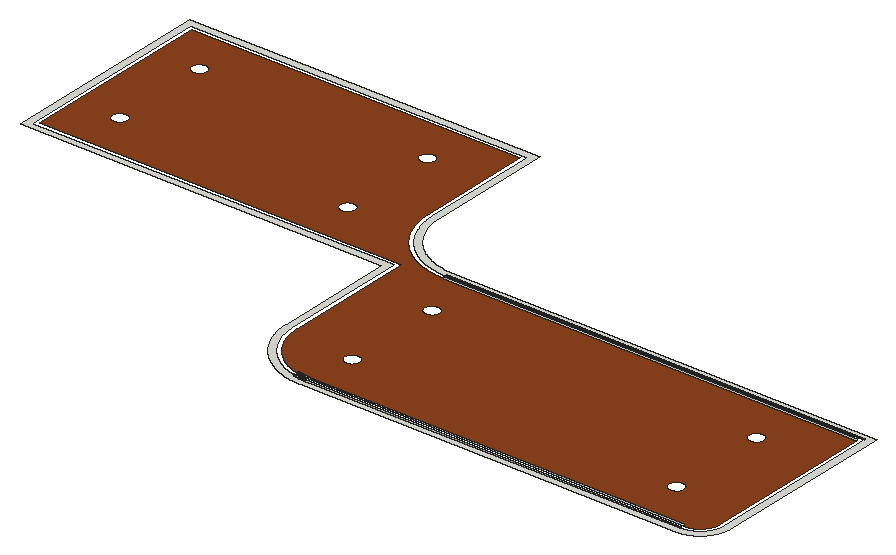
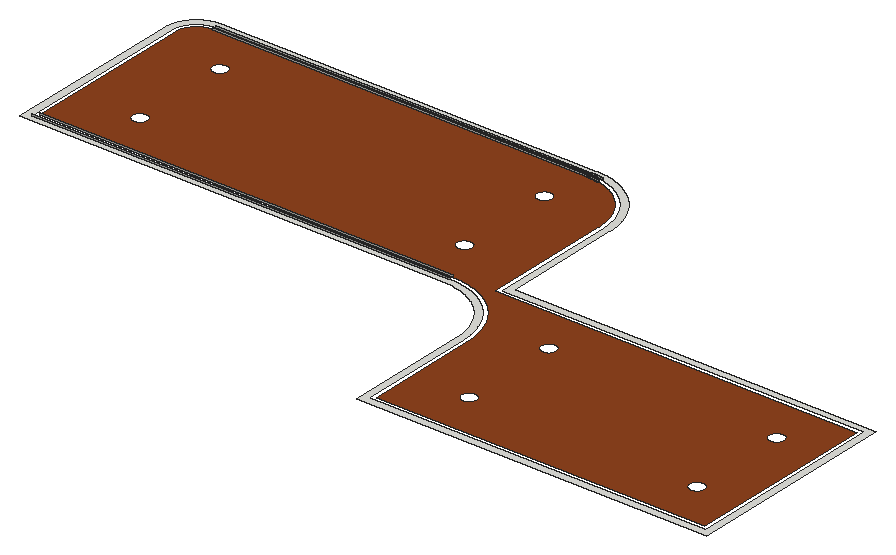
# SketchUp Ruby script. Lengths in inches.
U = 1.inch
M = Sketchup.active_model
def pt(a) = Geom::Point3d.new(a.map { |v| v * U })
def face(e, loops, mat)
  f = e.add_face(loops[0].map { |a| pt(a) })
  loops[1..].each { |l| e.add_face(l.map { |a| pt(a) }).erase! }
  f.material = f.back_material = mat if mat
  f
end
# faces: each face lists its corners as indices into pts; further lists are holes
def faces(e, pts, list, mat = nil) = list.each { |f| face(e, (f[0].is_a?(Array) ? f : [f]).map { |l| l.map { |i| pts[i] } }, mat) }
# xy, xz, yz: faces in a plane at the given z, y or x. An outline is a flat list of corners, or four numbers for a rectangle; further outlines are holes
def ring(l) = l.size == 4 ? [[l[0], l[1]], [l[2], l[1]], [l[2], l[3]], [l[0], l[3]]] : l.each_slice(2).to_a
def flat(e, list, mat, &to3) = list.each { |f| face(e, (f[0].is_a?(Array) ? f : [f]).map { |l| ring(l).map { |u, v| to3.(u, v) } }, mat) }
def xy(e, z, list, mat = nil) = flat(e, list, mat) { |x, y| [x, y, z] }
def xz(e, y, list, mat = nil) = flat(e, list, mat) { |x, z| [x, y, z] }
def yz(e, x, list, mat = nil) = flat(e, list, mat) { |y, z| [x, y, z] }
def lines(e, pts, list) = list.each { |a, b| e.add_line(pt(pts[a]), pt(pts[b])) }
# prism: a flat outline (further loops are holes) pulled along v
def prism(e, loops, v, mat = nil)
  f = face(e, loops, mat); d = Geom::Vector3d.new(v.map { |x| x * U })
  f.pushpull(f.normal.samedirection?(d) ? d.length : -d.length)
end
def box(e, o, s, mat = nil) = prism(e, [[o, [o[0] + s[0], o[1], o[2]], [o[0] + s[0], o[1] + s[1], o[2]], [o[0], o[1] + s[1], o[2]]]], [0, 0, s[2]], mat)
def at(x, y, z, deg = 0) = Geom::Transformation.translation(pt([x, y, z])) * Geom::Transformation.rotation(ORIGIN, Z_AXIS, deg.degrees)
def axes(o, x, y, z) = Geom::Transformation.new([*x, 0, *y, 0, *z, 0, *pt(o).to_a, 1])
def part(name) = M.definitions.add(name)
# library, detail: a bought-in or finely detailed component or shape, given as its bounding box
def library(name, o, s) = part(name).tap { |d| box(d.entities, o, s) }
def detail(e, o, s) = box(e.add_group.entities, o, s)
def put(e, d, t, mat = nil) = e.add_instance(d, t).tap { |i| i.material = mat if mat }
def group(e, t, mat = nil) = e.add_group.tap { |g| g.transformation = t; g.material = mat if mat }.entities
root = M.entities
M.materials.add("[Wood Fence]").color = [142, 67, 30]
xy(root,116,[[[157.71,122,157.42,122.01,157.14,122.02,156.85,122.03,156.5625,122.05,156.27,122.07,155.99,122.09,155.41,122.15,155.13,122.1875,154.84,122.23,154.56,122.27,154.27,122.32,153.71,122.42,153.43,122.48,153.14,122.54,152.58,122.68,152.31,122.75,151.75,122.91,151.48,122.99,151.2,123.08,150.66,123.26,150.12,123.46,149.85,123.57,149.58,123.67,149.32,123.79,149.05,123.9,148.53,124.14,148.01,124.4,147.76,124.53,147.5,124.67,146.75,125.09,146.51,125.24,146.26,125.39,145.3,126.03,144.84,126.37,144.61,126.55,144.38,126.72,144.15,126.9,143.93,127.09,143.71,127.27,143.49,127.46,143.07,127.84,142.44,128.44,141.84,129.07,141.46,129.49,141.27,129.71,141.09,129.93,140.9,130.15,140.72,130.38,140.55,130.61,140.37,130.84,140.03,131.3,139.39,132.26,139.24,132.51,139.09,132.75,138.67,133.5,138.53,133.76,138.4,134.01,138.14,134.53,137.9,135.05,137.79,135.32,137.67,135.58,137.57,135.85,137.46,136.12,137.26,136.66,137.08,137.2,136.99,137.48,136.91,137.75,136.75,138.31,136.68,138.58,136.54,139.14,136.48,139.43,136.42,139.71,136.32,140.27,136.27,140.56,136.23,140.84,136.1875,141.13,136.15,141.41,136.09,141.99,136.07,142.27,136.05,142.5625,136.03,142.85,136.02,143.14,136.01,143.42,136,143.71,136,182,20,182,20,250,132,250,132,209.76,132.01,209.52,132.01,209.28,132.02,209.03,132.04,208.79,132.05,208.55,132.09,208.07,132.21,207.11,132.33,206.39,132.37,206.16,132.47,205.68,132.52,205.45,132.58,205.21,132.7,204.75,132.77,204.51,133.05,203.59,133.13,203.36,133.22,203.13,133.3,202.91,133.39,202.68,133.48,202.46,133.57,202.23,133.66,202.01,133.86,201.57,133.97,201.35,134.07,201.14,134.18,200.92,134.29,200.71,134.4,200.49,134.88,199.65,135.01,199.45,135.14,199.24,135.4,198.84,135.82,198.24,135.96,198.05,136.71,197.1,137.35,196.38,137.52,196.2,137.6875,196.03,137.86,195.86,138.03,195.6875,138.2,195.52,138.38,195.35,139.1,194.71,140.05,193.96,140.24,193.82,140.84,193.4,141.24,193.14,141.45,193.01,141.65,192.88,142.49,192.4,142.71,192.29,142.92,192.18,143.14,192.07,143.35,191.97,143.57,191.86,144.01,191.66,144.23,191.57,144.46,191.48,144.68,191.39,144.91,191.3,145.13,191.22,145.36,191.13,145.59,191.05,146.51,190.77,146.75,190.7,147.21,190.58,147.45,190.52,147.68,190.47,148.16,190.37,148.39,190.33,149.11,190.21,150.07,190.09,150.55,190.05,150.79,190.04,151.03,190.02,151.28,190.01,151.52,190.01,151.76,190,288,190,288,131.8,287.99,131.61,287.98,131.41,287.97,131.22,287.93,130.82,287.91,130.63,287.875,130.4375,287.84,130.24,287.81,130.05,287.77,129.86,287.72,129.67,287.68,129.48,287.57,129.1,287.45,128.72,287.38,128.54,287.3125,128.36,287.24,128.17,287.16,127.99,287.08,127.8125,287,127.64,286.91,127.46,286.82,127.29,286.72,127.11,286.63,126.94,286.53,126.78,286.31,126.44,286.09,126.12,285.97,125.96,285.73,125.66,285.34,125.21,285.21,125.07,284.93,124.79,284.79,124.66,284.64,124.52,284.49,124.4,284.34,124.27,284.04,124.03,283.88,123.91,283.56,123.69,283.22,123.47,283.06,123.37,282.89,123.28,282.71,123.18,282.54,123.09,282.36,123,282.1875,122.92,282.01,122.84,281.83,122.76,281.64,122.6875,281.46,122.62,281.28,122.55,280.9,122.43,280.52,122.32,280.33,122.28,280.14,122.23,279.95,122.19,279.76,122.16,279.5625,122.125,279.37,122.09,279.18,122.07,278.78,122.03,278.59,122.02,278.39,122.01,278.2,122],[157.74,124,278.16,124,278.3125,124.01,278.47,124.01,278.63,124.02,278.78,124.04,279.1,124.08,279.25,124.1,279.41,124.125,279.5625,124.15,279.71,124.1875,279.87,124.22,280.32,124.34,280.77,124.49,280.92,124.55,281.0625,124.61,281.21,124.67,281.35,124.73,281.77,124.94,282.05,125.1,282.18,125.18,282.3125,125.26,282.44,125.35,282.57,125.4375,282.7,125.53,282.83,125.62,282.95,125.72,283.08,125.82,283.2,125.92,283.3125,126.02,283.43,126.125,283.54,126.23,283.66,126.34,283.77,126.46,283.875,126.57,283.98,126.6875,284.08,126.8,284.18,126.92,284.28,127.05,284.38,127.17,284.47,127.3,284.5625,127.43,284.65,127.56,284.74,127.6875,284.82,127.82,284.9,127.95,285.06,128.23,285.27,128.65,285.33,128.79,285.39,128.9375,285.45,129.08,285.51,129.23,285.66,129.68,285.78,130.13,285.8125,130.29,285.85,130.4375,285.875,130.59,285.9,130.75,285.92,130.9,285.96,131.22,285.98,131.37,285.99,131.53,285.99,131.6875,286,131.84,286,188,151.73,188,151.47,188.01,151.2,188.01,150.9375,188.03,150.67,188.04,150.41,188.06,150.14,188.08,149.875,188.1,149.61,188.13,149.35,188.16,149.08,188.19,148.56,188.27,148.3,188.3125,148.03,188.36,147.51,188.46,146.99,188.58,146.74,188.64,146.48,188.7,145.96,188.84,145.71,188.92,145.45,189,144.95,189.16,144.2,189.43,143.95,189.53,143.7,189.625,143.46,189.73,143.21,189.83,142.97,189.9375,142.73,190.05,142.49,190.16,142.01,190.4,141.78,190.52,141.54,190.64,141.08,190.9,140.85,191.04,140.62,191.17,140.39,191.3125,140.17,191.45,139.94,191.6,139.72,191.74,139.5,191.89,139.28,192.05,139.07,192.2,138.85,192.36,138.43,192.68,138.22,192.85,138.02,193.01,137.8125,193.18,137.61,193.36,137.41,193.53,137.21,193.71,137.02,193.89,136.82,194.07,136.63,194.26,136.44,194.44,136.26,194.63,136.07,194.82,135.89,195.02,135.71,195.21,135.53,195.41,135.36,195.61,135.18,195.8125,135.01,196.02,134.85,196.22,134.68,196.43,134.36,196.85,134.2,197.07,134.05,197.28,133.89,197.5,133.74,197.72,133.6,197.94,133.45,198.17,133.3125,198.39,133.17,198.62,133.04,198.85,132.9,199.08,132.64,199.54,132.52,199.78,132.4,200.01,132.16,200.49,132.05,200.73,131.9375,200.97,131.83,201.21,131.73,201.46,131.625,201.7,131.53,201.95,131.43,202.2,131.16,202.95,131,203.45,130.92,203.71,130.84,203.96,130.7,204.48,130.64,204.74,130.58,204.99,130.46,205.51,130.36,206.03,130.3125,206.3,130.27,206.56,130.19,207.08,130.16,207.35,130.13,207.61,130.1,207.875,130.08,208.14,130.06,208.41,130.04,208.67,130.03,208.9375,130.01,209.2,130.01,209.47,130,209.73,130,248,22,248,22,184,138,184,138,143.74,138.01,143.48,138.02,143.21,138.04,142.69,138.0625,142.43,138.08,142.17,138.17,141.39,138.29,140.61,138.33,140.36,138.38,140.1,138.4375,139.84,138.49,139.59,138.55,139.33,138.62,139.08,138.68,138.82,138.82,138.32,138.98,137.82,139.0625,137.57,139.15,137.32,139.24,137.08,139.33,136.83,139.42,136.59,139.52,136.35,139.73,135.87,139.84,135.625,139.95,135.39,140.0625,135.15,140.18,134.92,140.3,134.6875,140.42,134.46,140.68,134,140.8125,133.77,140.95,133.55,141.37,132.89,141.52,132.67,141.67,132.46,141.82,132.24,141.97,132.03,142.13,131.82,142.29,131.62,142.46,131.41,142.79,131.01,142.96,130.8125,143.14,130.62,143.3125,130.42,143.49,130.23,143.67,130.04,143.86,129.86,144.04,129.67,144.23,129.49,144.42,129.3125,144.62,129.14,144.8125,128.96,145.01,128.79,145.41,128.46,145.62,128.29,145.82,128.13,146.03,127.97,146.24,127.82,146.46,127.67,146.67,127.52,146.89,127.37,147.55,126.95,147.77,126.8125,148,126.68,148.46,126.42,148.6875,126.3,148.92,126.18,149.15,126.0625,149.39,125.95,149.625,125.84,149.87,125.73,150.35,125.52,150.59,125.42,150.83,125.33,151.08,125.24,151.32,125.15,151.57,125.0625,151.82,124.98,152.32,124.82,152.82,124.68,153.08,124.62,153.33,124.55,153.59,124.49,153.84,124.4375,154.1,124.38,154.36,124.33,154.61,124.29,155.39,124.17,156.17,124.08,156.43,124.0625,156.69,124.04,157.21,124.02,157.48,124.01]]])
xy(root,116,[[[157.76,125.5,157.52,125.51,157.27,125.51,157.03,125.53,156.79,125.54,156.07,125.6,155.35,125.69,154.63,125.81,154.39,125.86,154.15,125.9,153.92,125.96,153.68,126.01,153.45,126.07,153.21,126.13,152.98,126.19,152.75,126.26,152.51,126.33,152.28,126.41,152.05,126.48,151.82,126.5625,151.6,126.64,151.14,126.82,150.7,127,150.48,127.1,150.25,127.2,150.04,127.3,149.6,127.52,149.39,127.63,149.17,127.74,148.54,128.1,148.33,128.23,148.13,128.35,147.92,128.48,147.72,128.62,147.52,128.75,147.32,128.89,147.125,129.03,146.93,129.18,146.74,129.32,146.36,129.62,146.17,129.78,145.99,129.93,145.8,130.09,145.62,130.25,145.44,130.42,145.27,130.58,145.09,130.75,144.75,131.09,144.58,131.27,144.42,131.44,144.25,131.62,144.09,131.8,143.93,131.99,143.78,132.17,143.62,132.36,143.32,132.74,143.18,132.93,143.03,133.125,142.89,133.32,142.75,133.52,142.62,133.72,142.48,133.92,142.35,134.13,142.23,134.33,142.1,134.54,141.74,135.17,141.63,135.39,141.52,135.6,141.3,136.04,141.2,136.25,141.1,136.48,141,136.7,140.82,137.14,140.64,137.6,140.5625,137.82,140.48,138.05,140.41,138.28,140.33,138.51,140.26,138.75,140.19,138.98,140.13,139.21,140.07,139.45,140.01,139.68,139.96,139.92,139.9,140.15,139.86,140.39,139.81,140.63,139.69,141.35,139.6,142.07,139.54,142.79,139.53,143.03,139.51,143.27,139.51,143.52,139.5,143.76,139.5,185.5,23.5,185.5,23.5,246.5,128.5,246.5,128.5,209.72,128.51,209.43,128.52,209.15,128.53,208.86,128.54,208.58,128.5625,208.3,128.58,208.01,128.67,207.17,128.71,206.89,128.75,206.6,128.79,206.32,128.84,206.04,128.88,205.76,128.9375,205.49,128.99,205.21,129.05,204.93,129.12,204.65,129.18,204.375,129.25,204.1,129.33,203.83,129.4,203.55,129.48,203.28,129.5625,203.01,129.65,202.74,129.83,202.2,129.93,201.93,130.03,201.67,130.13,201.4,130.23,201.14,130.34,200.875,130.46,200.61,130.57,200.36,130.6875,200.1,130.81,199.84,130.93,199.58,131.0625,199.33,131.19,199.08,131.33,198.83,131.46,198.58,131.6,198.33,131.74,198.09,131.89,197.84,132.04,197.6,132.1875,197.36,132.34,197.12,132.5,196.89,132.66,196.65,132.82,196.42,132.99,196.1875,133.16,195.96,133.33,195.73,133.5,195.51,133.68,195.28,133.86,195.0625,134.04,194.85,134.22,194.63,134.79,194,134.99,193.79,135.18,193.58,135.58,193.18,135.79,192.99,136,192.79,136.63,192.22,136.85,192.04,137.0625,191.86,137.28,191.68,137.51,191.5,137.73,191.33,137.96,191.16,138.1875,190.99,138.42,190.82,138.65,190.66,138.89,190.5,139.12,190.34,139.36,190.1875,139.6,190.04,139.84,189.89,140.09,189.74,140.33,189.6,140.58,189.46,140.83,189.33,141.08,189.19,141.33,189.0625,141.58,188.93,141.84,188.81,142.1,188.6875,142.36,188.57,142.61,188.46,142.875,188.34,143.14,188.23,143.4,188.13,143.67,188.03,143.93,187.93,144.2,187.83,144.74,187.65,145.01,187.5625,145.28,187.48,145.55,187.4,145.83,187.33,146.1,187.25,146.375,187.18,146.65,187.12,146.93,187.05,147.21,186.99,147.49,186.9375,147.76,186.88,148.04,186.84,148.32,186.79,148.6,186.75,148.89,186.71,149.17,186.67,150.01,186.58,150.3,186.5625,150.58,186.54,150.86,186.53,151.15,186.52,151.71,186.5,284.5,186.5,284.5,131.87,284.49,131.74,284.49,131.62,284.47,131.36,284.45,131.24,284.4375,131.11,284.42,130.98,284.4,130.86,284.375,130.73,284.35,130.61,284.32,130.48,284.26,130.24,284.22,130.11,284.1,129.75,284.05,129.63,284.01,129.51,283.96,129.4,283.9,129.28,283.85,129.16,283.79,129.05,283.73,128.9375,283.67,128.82,283.61,128.71,283.54,128.6,283.47,128.5,283.33,128.28,283.26,128.18,283.1,127.98,283.02,127.875,282.94,127.78,282.86,127.68,282.77,127.59,282.69,127.49,282.6,127.4,282.5,127.3125,282.41,127.23,282.32,127.14,282.22,127.06,282.125,126.98,282.02,126.9,281.82,126.74,281.72,126.67,281.5,126.53,281.4,126.46,281.29,126.39,281.18,126.33,281.0625,126.27,280.95,126.21,280.84,126.15,280.72,126.1,280.6,126.04,280.49,125.99,280.37,125.95,280.25,125.9,279.89,125.78,279.76,125.74,279.52,125.68,279.39,125.65,279.27,125.625,279.14,125.6,279.02,125.58,278.89,125.5625,278.76,125.55,278.64,125.53,278.38,125.51,278.26,125.51,278.13,125.5],[159.84,137.5,160.16,137.5,160.24,137.51,160.3125,137.52,160.39,137.53,160.47,137.54,160.55,137.56,160.62,137.58,160.7,137.6,160.77,137.62,160.85,137.65,160.99,137.71,161.0625,137.74,161.13,137.77,161.41,137.93,161.47,137.98,161.53,138.02,161.59,138.07,161.71,138.18,161.77,138.23,161.82,138.29,161.93,138.41,161.98,138.47,162.02,138.53,162.07,138.59,162.23,138.87,162.26,138.9375,162.29,139.01,162.35,139.15,162.38,139.23,162.4,139.3,162.42,139.38,162.44,139.45,162.46,139.53,162.47,139.61,162.48,139.6875,162.49,139.76,162.5,139.84,162.5,140.16,162.49,140.24,162.48,140.3125,162.47,140.39,162.46,140.47,162.44,140.55,162.42,140.62,162.4,140.7,162.38,140.77,162.35,140.85,162.29,140.99,162.26,141.0625,162.23,141.13,162.07,141.41,162.02,141.47,161.98,141.53,161.93,141.59,161.82,141.71,161.77,141.77,161.71,141.82,161.59,141.93,161.53,141.98,161.47,142.02,161.41,142.07,161.13,142.23,161.0625,142.26,160.99,142.29,160.85,142.35,160.77,142.38,160.7,142.4,160.62,142.42,160.55,142.44,160.47,142.46,160.39,142.47,160.3125,142.48,160.24,142.49,160.16,142.5,159.84,142.5,159.76,142.49,159.6875,142.48,159.61,142.47,159.53,142.46,159.45,142.44,159.38,142.42,159.3,142.4,159.23,142.38,159.15,142.35,159.01,142.29,158.9375,142.26,158.87,142.23,158.59,142.07,158.53,142.02,158.47,141.98,158.41,141.93,158.29,141.82,158.23,141.77,158.18,141.71,158.07,141.59,158.02,141.53,157.98,141.47,157.93,141.41,157.77,141.13,157.74,141.0625,157.71,140.99,157.65,140.85,157.62,140.77,157.6,140.7,157.58,140.62,157.56,140.55,157.54,140.47,157.53,140.39,157.52,140.3125,157.51,140.24,157.5,140.16,157.5,139.84,157.51,139.76,157.52,139.6875,157.53,139.61,157.54,139.53,157.56,139.45,157.58,139.38,157.6,139.3,157.62,139.23,157.65,139.15,157.71,139.01,157.74,138.9375,157.77,138.87,157.93,138.59,157.98,138.53,158.02,138.47,158.07,138.41,158.18,138.29,158.23,138.23,158.29,138.18,158.41,138.07,158.47,138.02,158.53,137.98,158.59,137.93,158.87,137.77,158.9375,137.74,159.01,137.71,159.15,137.65,159.23,137.62,159.3,137.6,159.38,137.58,159.45,137.56,159.53,137.54,159.61,137.53,159.6875,137.52,159.76,137.51],[37.34,197.5,37.66,197.5,37.74,197.51,37.8125,197.52,37.89,197.53,37.97,197.54,38.05,197.56,38.12,197.58,38.2,197.6,38.27,197.62,38.35,197.65,38.49,197.71,38.5625,197.74,38.63,197.77,38.91,197.93,38.97,197.98,39.03,198.02,39.09,198.07,39.21,198.18,39.27,198.23,39.32,198.29,39.43,198.41,39.48,198.47,39.52,198.53,39.57,198.59,39.73,198.87,39.76,198.9375,39.79,199.01,39.85,199.15,39.88,199.23,39.9,199.3,39.92,199.38,39.94,199.45,39.96,199.53,39.97,199.61,39.98,199.6875,39.99,199.76,40,199.84,40,200.16,39.99,200.24,39.98,200.3125,39.97,200.39,39.96,200.47,39.94,200.55,39.92,200.62,39.9,200.7,39.88,200.77,39.85,200.85,39.79,200.99,39.76,201.0625,39.73,201.13,39.57,201.41,39.52,201.47,39.48,201.53,39.43,201.59,39.32,201.71,39.27,201.77,39.21,201.82,39.09,201.93,39.03,201.98,38.97,202.02,38.91,202.07,38.63,202.23,38.5625,202.26,38.49,202.29,38.35,202.35,38.27,202.38,38.2,202.4,38.12,202.42,38.05,202.44,37.97,202.46,37.89,202.47,37.8125,202.48,37.74,202.49,37.66,202.5,37.34,202.5,37.26,202.49,37.1875,202.48,37.11,202.47,37.03,202.46,36.95,202.44,36.88,202.42,36.8,202.4,36.73,202.38,36.65,202.35,36.51,202.29,36.4375,202.26,36.37,202.23,36.09,202.07,36.03,202.02,35.97,201.98,35.91,201.93,35.79,201.82,35.73,201.77,35.68,201.71,35.57,201.59,35.52,201.53,35.48,201.47,35.43,201.41,35.27,201.13,35.24,201.0625,35.21,200.99,35.15,200.85,35.12,200.77,35.1,200.7,35.08,200.62,35.06,200.55,35.04,200.47,35.03,200.39,35.02,200.3125,35.01,200.24,35,200.16,35,199.84,35.01,199.76,35.02,199.6875,35.03,199.61,35.04,199.53,35.06,199.45,35.08,199.38,35.1,199.3,35.12,199.23,35.15,199.15,35.21,199.01,35.24,198.9375,35.27,198.87,35.43,198.59,35.48,198.53,35.52,198.47,35.57,198.41,35.68,198.29,35.73,198.23,35.79,198.18,35.91,198.07,35.97,198.02,36.03,197.98,36.09,197.93,36.37,197.77,36.4375,197.74,36.51,197.71,36.65,197.65,36.73,197.62,36.8,197.6,36.88,197.58,36.95,197.56,37.03,197.54,37.11,197.53,37.1875,197.52,37.26,197.51],[159.84,169.5,160.16,169.5,160.24,169.51,160.3125,169.52,160.39,169.53,160.47,169.54,160.55,169.56,160.62,169.58,160.7,169.6,160.77,169.62,160.85,169.65,160.99,169.71,161.0625,169.74,161.13,169.77,161.41,169.93,161.47,169.98,161.53,170.02,161.59,170.07,161.71,170.18,161.77,170.23,161.82,170.29,161.93,170.41,161.98,170.47,162.02,170.53,162.07,170.59,162.23,170.87,162.26,170.9375,162.29,171.01,162.35,171.15,162.38,171.23,162.4,171.3,162.42,171.38,162.44,171.45,162.46,171.53,162.47,171.61,162.48,171.6875,162.49,171.76,162.5,171.84,162.5,172.16,162.49,172.24,162.48,172.3125,162.47,172.39,162.46,172.47,162.44,172.55,162.42,172.62,162.4,172.7,162.38,172.77,162.35,172.85,162.29,172.99,162.26,173.0625,162.23,173.13,162.07,173.41,162.02,173.47,161.98,173.53,161.93,173.59,161.82,173.71,161.77,173.77,161.71,173.82,161.59,173.93,161.53,173.98,161.47,174.02,161.41,174.07,161.13,174.23,161.0625,174.26,160.99,174.29,160.85,174.35,160.77,174.38,160.7,174.4,160.62,174.42,160.55,174.44,160.47,174.46,160.39,174.47,160.3125,174.48,160.24,174.49,160.16,174.5,159.84,174.5,159.76,174.49,159.6875,174.48,159.61,174.47,159.53,174.46,159.45,174.44,159.38,174.42,159.3,174.4,159.23,174.38,159.15,174.35,159.01,174.29,158.9375,174.26,158.87,174.23,158.59,174.07,158.53,174.02,158.47,173.98,158.41,173.93,158.29,173.82,158.23,173.77,158.18,173.71,158.07,173.59,158.02,173.53,157.98,173.47,157.93,173.41,157.77,173.13,157.74,173.0625,157.71,172.99,157.65,172.85,157.62,172.77,157.6,172.7,157.58,172.62,157.56,172.55,157.54,172.47,157.53,172.39,157.52,172.3125,157.51,172.24,157.5,172.16,157.5,171.84,157.51,171.76,157.52,171.6875,157.53,171.61,157.54,171.53,157.56,171.45,157.58,171.38,157.6,171.3,157.62,171.23,157.65,171.15,157.71,171.01,157.74,170.9375,157.77,170.87,157.93,170.59,157.98,170.53,158.02,170.47,158.07,170.41,158.18,170.29,158.23,170.23,158.29,170.18,158.41,170.07,158.47,170.02,158.53,169.98,158.59,169.93,158.87,169.77,158.9375,169.74,159.01,169.71,159.15,169.65,159.23,169.62,159.3,169.6,159.38,169.58,159.45,169.56,159.53,169.54,159.61,169.53,159.6875,169.52,159.76,169.51],[110.34,229.5,110.66,229.5,110.74,229.51,110.8125,229.52,110.89,229.53,110.97,229.54,111.05,229.56,111.12,229.58,111.2,229.6,111.27,229.62,111.35,229.65,111.49,229.71,111.5625,229.74,111.63,229.77,111.91,229.93,111.97,229.98,112.03,230.02,112.09,230.07,112.21,230.18,112.27,230.23,112.32,230.29,112.43,230.41,112.48,230.47,112.52,230.53,112.57,230.59,112.73,230.87,112.76,230.9375,112.79,231.01,112.85,231.15,112.88,231.23,112.9,231.3,112.92,231.38,112.94,231.45,112.96,231.53,112.97,231.61,112.98,231.6875,112.99,231.76,113,231.84,113,232.16,112.99,232.24,112.98,232.3125,112.97,232.39,112.96,232.47,112.94,232.55,112.92,232.62,112.9,232.7,112.88,232.77,112.85,232.85,112.79,232.99,112.76,233.0625,112.73,233.13,112.57,233.41,112.52,233.47,112.48,233.53,112.43,233.59,112.32,233.71,112.27,233.77,112.21,233.82,112.09,233.93,112.03,233.98,111.97,234.02,111.91,234.07,111.63,234.23,111.5625,234.26,111.49,234.29,111.35,234.35,111.27,234.38,111.2,234.4,111.12,234.42,111.05,234.44,110.97,234.46,110.89,234.47,110.8125,234.48,110.74,234.49,110.66,234.5,110.34,234.5,110.26,234.49,110.1875,234.48,110.11,234.47,110.03,234.46,109.95,234.44,109.88,234.42,109.8,234.4,109.73,234.38,109.65,234.35,109.51,234.29,109.4375,234.26,109.37,234.23,109.09,234.07,109.03,234.02,108.97,233.98,108.91,233.93,108.79,233.82,108.73,233.77,108.68,233.71,108.57,233.59,108.52,233.53,108.48,233.47,108.43,233.41,108.27,233.13,108.24,233.0625,108.21,232.99,108.15,232.85,108.12,232.77,108.1,232.7,108.08,232.62,108.06,232.55,108.04,232.47,108.03,232.39,108.02,232.3125,108.01,232.24,108,232.16,108,231.84,108.01,231.76,108.02,231.6875,108.03,231.61,108.04,231.53,108.06,231.45,108.08,231.38,108.1,231.3,108.12,231.23,108.15,231.15,108.21,231.01,108.24,230.9375,108.27,230.87,108.43,230.59,108.48,230.53,108.52,230.47,108.57,230.41,108.68,230.29,108.73,230.23,108.79,230.18,108.91,230.07,108.97,230.02,109.03,229.98,109.09,229.93,109.37,229.77,109.4375,229.74,109.51,229.71,109.65,229.65,109.73,229.62,109.8,229.6,109.88,229.58,109.95,229.56,110.03,229.54,110.11,229.53,110.1875,229.52,110.26,229.51],[110.34,197.5,110.66,197.5,110.74,197.51,110.8125,197.52,110.89,197.53,110.97,197.54,111.05,197.56,111.12,197.58,111.2,197.6,111.27,197.62,111.35,197.65,111.49,197.71,111.5625,197.74,111.63,197.77,111.91,197.93,111.97,197.98,112.03,198.02,112.09,198.07,112.21,198.18,112.27,198.23,112.32,198.29,112.43,198.41,112.48,198.47,112.52,198.53,112.57,198.59,112.73,198.87,112.76,198.9375,112.79,199.01,112.85,199.15,112.88,199.23,112.9,199.3,112.92,199.38,112.94,199.45,112.96,199.53,112.97,199.61,112.98,199.6875,112.99,199.76,113,199.84,113,200.16,112.99,200.24,112.98,200.3125,112.97,200.39,112.96,200.47,112.94,200.55,112.92,200.62,112.9,200.7,112.88,200.77,112.85,200.85,112.79,200.99,112.76,201.0625,112.73,201.13,112.57,201.41,112.52,201.47,112.48,201.53,112.43,201.59,112.32,201.71,112.27,201.77,112.21,201.82,112.09,201.93,112.03,201.98,111.97,202.02,111.91,202.07,111.63,202.23,111.5625,202.26,111.49,202.29,111.35,202.35,111.27,202.38,111.2,202.4,111.12,202.42,111.05,202.44,110.97,202.46,110.89,202.47,110.8125,202.48,110.74,202.49,110.66,202.5,110.34,202.5,110.26,202.49,110.1875,202.48,110.11,202.47,110.03,202.46,109.95,202.44,109.88,202.42,109.8,202.4,109.73,202.38,109.65,202.35,109.51,202.29,109.4375,202.26,109.37,202.23,109.09,202.07,109.03,202.02,108.97,201.98,108.91,201.93,108.79,201.82,108.73,201.77,108.68,201.71,108.57,201.59,108.52,201.53,108.48,201.47,108.43,201.41,108.27,201.13,108.24,201.0625,108.21,200.99,108.15,200.85,108.12,200.77,108.1,200.7,108.08,200.62,108.06,200.55,108.04,200.47,108.03,200.39,108.02,200.3125,108.01,200.24,108,200.16,108,199.84,108.01,199.76,108.02,199.6875,108.03,199.61,108.04,199.53,108.06,199.45,108.08,199.38,108.1,199.3,108.12,199.23,108.15,199.15,108.21,199.01,108.24,198.9375,108.27,198.87,108.43,198.59,108.48,198.53,108.52,198.47,108.57,198.41,108.68,198.29,108.73,198.23,108.79,198.18,108.91,198.07,108.97,198.02,109.03,197.98,109.09,197.93,109.37,197.77,109.4375,197.74,109.51,197.71,109.65,197.65,109.73,197.62,109.8,197.6,109.88,197.58,109.95,197.56,110.03,197.54,110.11,197.53,110.1875,197.52,110.26,197.51],[263.84,169.5,264.16,169.5,264.24,169.51,264.3125,169.52,264.39,169.53,264.47,169.54,264.55,169.56,264.62,169.58,264.7,169.6,264.77,169.62,264.85,169.65,264.99,169.71,265.0625,169.74,265.13,169.77,265.41,169.93,265.47,169.98,265.53,170.02,265.59,170.07,265.71,170.18,265.77,170.23,265.82,170.29,265.93,170.41,265.98,170.47,266.02,170.53,266.07,170.59,266.23,170.87,266.26,170.9375,266.29,171.01,266.35,171.15,266.38,171.23,266.4,171.3,266.42,171.38,266.44,171.45,266.46,171.53,266.47,171.61,266.48,171.6875,266.49,171.76,266.49,171.84,266.5,171.92,266.5,172.08,266.49,172.16,266.49,172.24,266.48,172.3125,266.47,172.39,266.46,172.47,266.44,172.55,266.42,172.62,266.4,172.7,266.38,172.77,266.35,172.85,266.29,172.99,266.26,173.0625,266.23,173.13,266.07,173.41,266.02,173.47,265.98,173.53,265.93,173.59,265.82,173.71,265.77,173.77,265.71,173.82,265.59,173.93,265.53,173.98,265.47,174.02,265.41,174.07,265.13,174.23,265.0625,174.26,264.99,174.29,264.85,174.35,264.77,174.38,264.7,174.4,264.62,174.42,264.55,174.44,264.47,174.46,264.39,174.47,264.3125,174.48,264.24,174.49,264.16,174.5,263.84,174.5,263.76,174.49,263.6875,174.48,263.61,174.47,263.53,174.46,263.45,174.44,263.38,174.42,263.3,174.4,263.23,174.38,263.15,174.35,262.94,174.26,262.86,174.23,262.8,174.19,262.59,174.07,262.53,174.02,262.47,173.98,262.41,173.93,262.29,173.82,262.23,173.77,262.18,173.71,262.07,173.59,262.02,173.53,261.98,173.47,261.93,173.41,261.77,173.13,261.74,173.0625,261.71,172.99,261.65,172.85,261.62,172.77,261.6,172.7,261.58,172.62,261.56,172.55,261.54,172.47,261.53,172.39,261.52,172.3125,261.51,172.24,261.5,172.16,261.5,171.84,261.51,171.76,261.52,171.6875,261.53,171.61,261.54,171.53,261.56,171.45,261.58,171.38,261.6,171.3,261.62,171.23,261.65,171.15,261.71,171.01,261.74,170.9375,261.77,170.87,261.93,170.59,261.98,170.53,262.02,170.47,262.07,170.41,262.18,170.29,262.23,170.23,262.29,170.18,262.41,170.07,262.47,170.02,262.53,169.98,262.59,169.93,262.8,169.81,262.86,169.77,262.94,169.74,263.15,169.65,263.23,169.62,263.3,169.6,263.38,169.58,263.45,169.56,263.53,169.54,263.61,169.53,263.6875,169.52,263.76,169.51],[263.84,137.5,264.16,137.5,264.24,137.51,264.3125,137.52,264.39,137.53,264.47,137.54,264.55,137.56,264.62,137.58,264.7,137.6,264.77,137.62,264.85,137.65,264.99,137.71,265.0625,137.74,265.13,137.77,265.41,137.93,265.47,137.98,265.53,138.02,265.59,138.07,265.71,138.18,265.77,138.23,265.82,138.29,265.93,138.41,265.98,138.47,266.02,138.53,266.07,138.59,266.23,138.87,266.26,138.9375,266.29,139.01,266.35,139.15,266.38,139.23,266.4,139.3,266.42,139.38,266.44,139.45,266.46,139.53,266.47,139.61,266.48,139.6875,266.49,139.76,266.49,139.84,266.5,139.92,266.5,140.08,266.49,140.16,266.49,140.24,266.48,140.3125,266.47,140.39,266.46,140.47,266.44,140.55,266.42,140.62,266.4,140.7,266.38,140.77,266.35,140.85,266.29,140.99,266.26,141.0625,266.23,141.13,266.07,141.41,266.02,141.47,265.98,141.53,265.93,141.59,265.82,141.71,265.77,141.77,265.71,141.82,265.59,141.93,265.53,141.98,265.47,142.02,265.41,142.07,265.13,142.23,265.0625,142.26,264.99,142.29,264.85,142.35,264.77,142.38,264.7,142.4,264.62,142.42,264.55,142.44,264.47,142.46,264.39,142.47,264.3125,142.48,264.24,142.49,264.16,142.5,263.84,142.5,263.76,142.49,263.6875,142.48,263.61,142.47,263.53,142.46,263.45,142.44,263.38,142.42,263.3,142.4,263.23,142.38,263.15,142.35,262.94,142.26,262.86,142.23,262.8,142.19,262.59,142.07,262.53,142.02,262.47,141.98,262.41,141.93,262.29,141.82,262.23,141.77,262.18,141.71,262.07,141.59,262.02,141.53,261.98,141.47,261.93,141.41,261.77,141.13,261.74,141.0625,261.71,140.99,261.65,140.85,261.62,140.77,261.6,140.7,261.58,140.62,261.56,140.55,261.54,140.47,261.53,140.39,261.52,140.3125,261.51,140.24,261.5,140.16,261.5,139.84,261.51,139.76,261.52,139.6875,261.53,139.61,261.54,139.53,261.56,139.45,261.58,139.38,261.6,139.3,261.62,139.23,261.65,139.15,261.71,139.01,261.74,138.9375,261.77,138.87,261.93,138.59,261.98,138.53,262.02,138.47,262.07,138.41,262.18,138.29,262.23,138.23,262.29,138.18,262.41,138.07,262.47,138.02,262.53,137.98,262.59,137.93,262.8,137.81,262.86,137.77,262.94,137.74,263.15,137.65,263.23,137.62,263.3,137.6,263.38,137.58,263.45,137.56,263.53,137.54,263.61,137.53,263.6875,137.52,263.76,137.51],[37.34,229.5,37.66,229.5,37.74,229.51,37.8125,229.52,37.89,229.53,37.97,229.54,38.05,229.56,38.12,229.58,38.2,229.6,38.27,229.62,38.35,229.65,38.49,229.71,38.5625,229.74,38.63,229.77,38.91,229.93,38.97,229.98,39.03,230.02,39.09,230.07,39.21,230.18,39.27,230.23,39.32,230.29,39.43,230.41,39.48,230.47,39.52,230.53,39.57,230.59,39.73,230.87,39.76,230.9375,39.79,231.01,39.85,231.15,39.88,231.23,39.9,231.3,39.92,231.38,39.94,231.45,39.96,231.53,39.97,231.61,39.98,231.6875,39.99,231.76,40,231.84,40,232.16,39.99,232.24,39.98,232.3125,39.97,232.39,39.96,232.47,39.94,232.55,39.92,232.62,39.9,232.7,39.88,232.77,39.85,232.85,39.79,232.99,39.76,233.0625,39.73,233.13,39.57,233.41,39.52,233.47,39.48,233.53,39.43,233.59,39.32,233.71,39.27,233.77,39.21,233.82,39.09,233.93,39.03,233.98,38.97,234.02,38.91,234.07,38.63,234.23,38.5625,234.26,38.49,234.29,38.35,234.35,38.27,234.38,38.2,234.4,38.12,234.42,38.05,234.44,37.97,234.46,37.89,234.47,37.8125,234.48,37.74,234.49,37.66,234.5,37.34,234.5,37.26,234.49,37.1875,234.48,37.11,234.47,37.03,234.46,36.95,234.44,36.88,234.42,36.8,234.4,36.73,234.38,36.65,234.35,36.51,234.29,36.4375,234.26,36.37,234.23,36.09,234.07,36.03,234.02,35.97,233.98,35.91,233.93,35.79,233.82,35.73,233.77,35.68,233.71,35.57,233.59,35.52,233.53,35.48,233.47,35.43,233.41,35.27,233.13,35.24,233.0625,35.21,232.99,35.15,232.85,35.12,232.77,35.1,232.7,35.08,232.62,35.06,232.55,35.04,232.47,35.03,232.39,35.02,232.3125,35.01,232.24,35,232.16,35,231.84,35.01,231.76,35.02,231.6875,35.03,231.61,35.04,231.53,35.06,231.45,35.08,231.38,35.1,231.3,35.12,231.23,35.15,231.15,35.21,231.01,35.24,230.9375,35.27,230.87,35.43,230.59,35.48,230.53,35.52,230.47,35.57,230.41,35.68,230.29,35.73,230.23,35.79,230.18,35.91,230.07,35.97,230.02,36.03,229.98,36.09,229.93,36.37,229.77,36.4375,229.74,36.51,229.71,36.65,229.65,36.73,229.62,36.8,229.6,36.88,229.58,36.95,229.56,37.03,229.54,37.11,229.53,37.1875,229.52,37.26,229.51]]],"[Wood Fence]")
xz(root,124,[[157.74,116,158,116.5],[158,116,278,116.5]])
xz(root,125.5,[[157.76,116,158,116.5],[158,116,278,116.5]])
xz(root,125.51,[[157.27,116,157.52,116.5]])
xz(root,186.5,[[152,116,284.5,116.5]])
xz(root,188,[[152,116,286,116.5]])
p = [[156.69,124.04,116],[156.43,124.0625,116],[156.43,124.0625,116.5],[156.69,124.04,116.5],[156.95,124.03,116],[156.95,124.03,116.5],
  [157.21,124.02,116],[157.21,124.02,116.5],[157.48,124.01,116],[157.48,124.01,116.5],[157.74,124,116],[157.74,124,116.5],
  [155.65,124.14,116],[155.39,124.17,116],[155.39,124.17,116.5],[155.65,124.14,116.5],[155.91,124.11,116],[155.91,124.11,116.5],
  [156.17,124.08,116],[156.17,124.08,116.5],[154.87,124.25,116],[154.61,124.29,116],[154.61,124.29,116.5],[154.87,124.25,116.5],
  [155.13,124.21,116],[155.13,124.21,116.5],[154.36,124.33,116],[154.1,124.38,116],[154.1,124.38,116.5],[154.36,124.33,116.5],
  [153.84,124.4375,116],[153.59,124.49,116],[153.59,124.49,116.5],[153.84,124.4375,116.5],[156.55,125.56,116],[156.79,125.54,116],
  [156.79,125.54,116.5],[156.55,125.56,116.5],[157.03,125.53,116],[157.03,125.53,116.5],[157.27,125.51,116],[157.27,125.51,116.5],
  [157.52,125.51,116],[157.76,125.5,116],[157.76,125.5,116.5],[157.52,125.51,116.5],[155.59,125.66,116],[155.83,125.63,116],
  [155.83,125.63,116.5],[155.59,125.66,116.5],[156.07,125.6,116],[156.07,125.6,116.5],[156.31,125.58,116],[156.31,125.58,116.5],
  [154.87,125.77,116],[155.11,125.73,116],[155.11,125.73,116.5],[154.87,125.77,116.5],[155.35,125.69,116],[155.35,125.69,116.5],
  [154.39,125.86,116],[154.63,125.81,116],[154.63,125.81,116.5],[154.39,125.86,116.5],[153.92,125.96,116],[154.15,125.9,116],
  [154.15,125.9,116.5],[153.92,125.96,116.5],[153.68,126.01,116],[153.68,126.01,116.5]]
faces(root,p,[[0,1,2,3],[4,0,3,5],[6,4,5,7],[8,6,7,9],[10,8,9,11],[12,13,14,15],[16,12,15,17],[18,16,17,19],
  [1,18,19,2],[20,21,22,23],[24,20,23,25],[13,24,25,14],[26,27,28,29],[21,26,29,22],[30,31,32,33],[27,30,33,28],
  [34,35,36,37],[35,38,39,36],[38,40,41,39],[42,43,44,45],[46,47,48,49],[47,50,51,48],[50,52,53,51],[52,34,37,53],
  [54,55,56,57],[55,58,59,56],[58,46,49,59],[60,61,62,63],[61,54,57,62],[64,65,66,67],[65,60,63,66],[68,64,67,69]])
